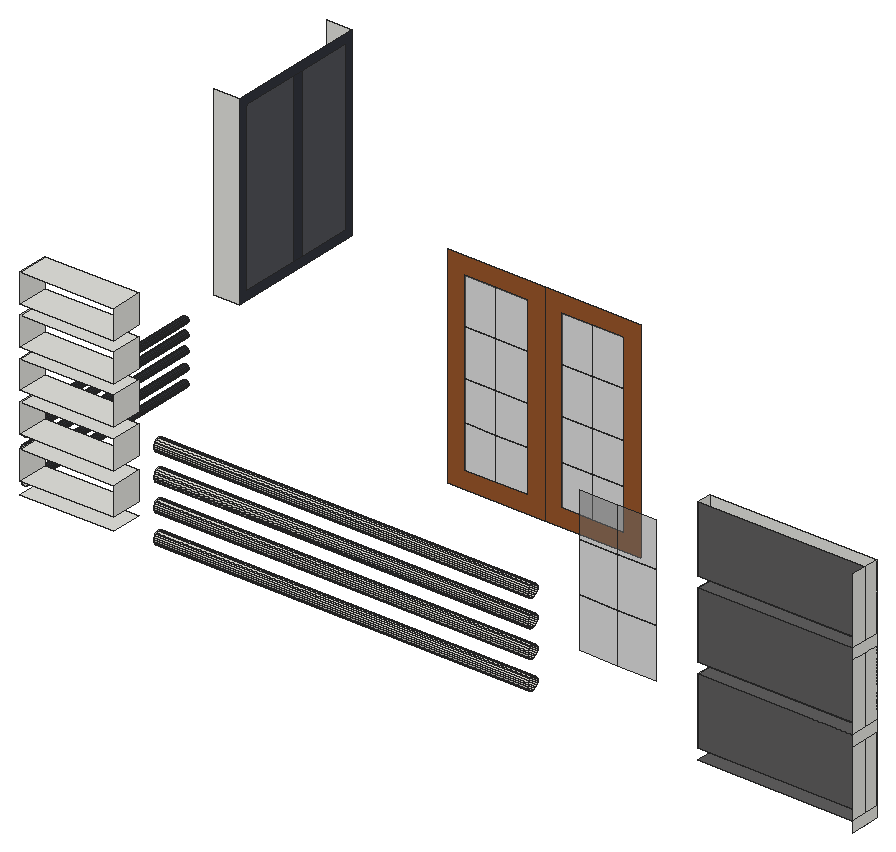
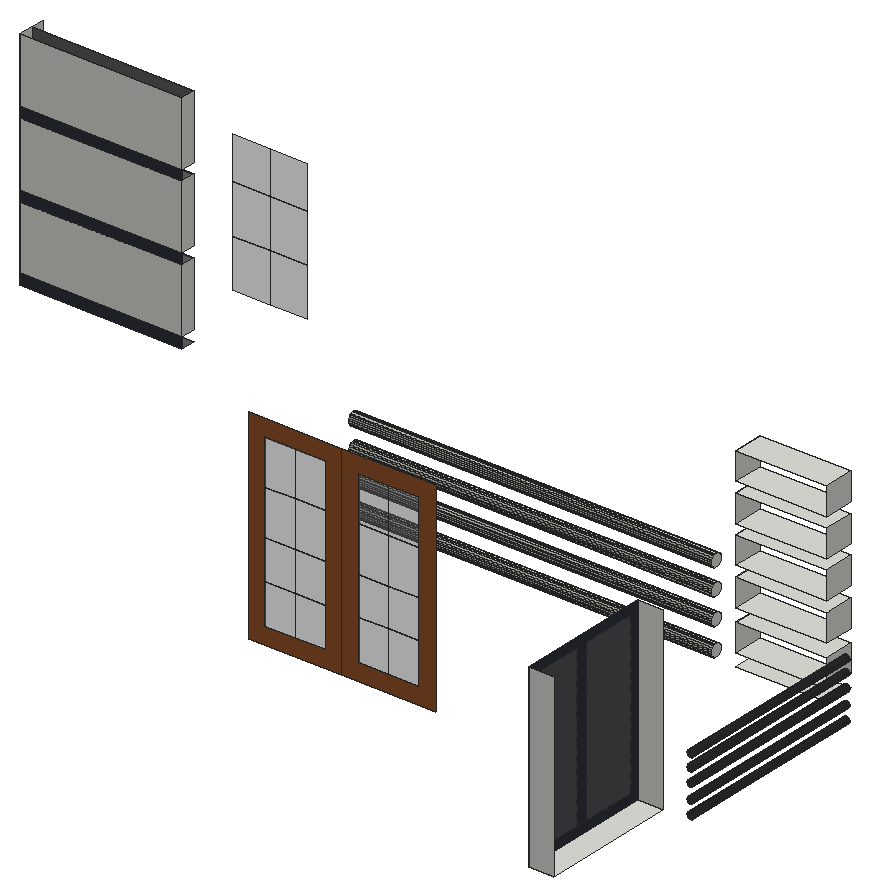
# SketchUp Ruby script. Lengths in inches.
U = 1.inch
M = Sketchup.active_model
def pt(a) = Geom::Point3d.new(a.map { |v| v * U })
def face(e, loops, mat)
  f = e.add_face(loops[0].map { |a| pt(a) })
  loops[1..].each { |l| e.add_face(l.map { |a| pt(a) }).erase! }
  f.material = f.back_material = mat if mat
  f
end
# faces: each face lists its corners as indices into pts; further lists are holes
def faces(e, pts, list, mat = nil) = list.each { |f| face(e, (f[0].is_a?(Array) ? f : [f]).map { |l| l.map { |i| pts[i] } }, mat) }
# xy, xz, yz: faces in a plane at the given z, y or x. An outline is a flat list of corners, or four numbers for a rectangle; further outlines are holes
def ring(l) = l.size == 4 ? [[l[0], l[1]], [l[2], l[1]], [l[2], l[3]], [l[0], l[3]]] : l.each_slice(2).to_a
def flat(e, list, mat, &to3) = list.each { |f| face(e, (f[0].is_a?(Array) ? f : [f]).map { |l| ring(l).map { |u, v| to3.(u, v) } }, mat) }
def xy(e, z, list, mat = nil) = flat(e, list, mat) { |x, y| [x, y, z] }
def xz(e, y, list, mat = nil) = flat(e, list, mat) { |x, z| [x, y, z] }
def yz(e, x, list, mat = nil) = flat(e, list, mat) { |y, z| [x, y, z] }
def lines(e, pts, list) = list.each { |a, b| e.add_line(pt(pts[a]), pt(pts[b])) }
# prism: a flat outline (further loops are holes) pulled along v
def prism(e, loops, v, mat = nil)
  f = face(e, loops, mat); d = Geom::Vector3d.new(v.map { |x| x * U })
  f.pushpull(f.normal.samedirection?(d) ? d.length : -d.length)
end
def box(e, o, s, mat = nil) = prism(e, [[o, [o[0] + s[0], o[1], o[2]], [o[0] + s[0], o[1] + s[1], o[2]], [o[0], o[1] + s[1], o[2]]]], [0, 0, s[2]], mat)
def at(x, y, z, deg = 0) = Geom::Transformation.translation(pt([x, y, z])) * Geom::Transformation.rotation(ORIGIN, Z_AXIS, deg.degrees)
def axes(o, x, y, z) = Geom::Transformation.new([*x, 0, *y, 0, *z, 0, *pt(o).to_a, 1])
def part(name) = M.definitions.add(name)
# library, detail: a bought-in or finely detailed component or shape, given as its bounding box
def library(name, o, s) = part(name).tap { |d| box(d.entities, o, s) }
def detail(e, o, s) = box(e.add_group.entities, o, s)
def put(e, d, t, mat = nil) = e.add_instance(d, t).tap { |i| i.material = mat if mat }
def group(e, t, mat = nil) = e.add_group.tap { |g| g.transformation = t; g.material = mat if mat }.entities
root = M.entities
M.materials.add("[Blinds Roman Hobbled Blue]").color = [81, 82, 87]
M.materials.add("[Formica Laminate Dark]").color = [50, 53, 60]
M.materials.add("[Granite Dark Gray]").color = [96, 95, 95]
M.materials.add("[Terrazzo Tile Light]").color = [219, 217, 210]
M.materials.add("[Translucent Glass Gray]").color = [128, 128, 128]
M.materials["[Translucent Glass Gray]"].alpha = 0.5
M.materials.add("[Wood Cherry Original]").color = [152, 86, 42]
xy(root,221.9,[[23.59,55.96,54.34,66.17]])
xy(root,226.03,[[23.59,55.96,54.34,66.17]])
xy(root,232.83,[[9.125,153.59,17.5,199.9]])
xy(root,235.3125,[[261.16,37.37,315.98,42.24]],"[Granite Dark Gray]")
xy(root,235.4,[[23.59,55.96,54.34,66.17]])
xy(root,238.87,[[261.16,37.37,315.98,42.24]],"[Granite Dark Gray]")
xy(root,239.78,[[23.59,55.96,54.34,66.17]])
xy(root,249.15,[[23.59,55.96,54.34,66.17]])
xy(root,252.65,[[23.59,55.96,54.34,66.17]])
xy(root,260.6875,[[261.16,37.37,315.98,42.24]],"[Granite Dark Gray]")
xy(root,262.03,[[23.59,55.96,54.34,66.17]])
xy(root,264.24,[[261.16,37.37,315.98,42.24]],"[Granite Dark Gray]")
xy(root,265.34,[[23.59,55.96,54.34,66.17]])
xy(root,274.72,[[23.59,55.96,54.34,66.17]])
xy(root,278.15,[[23.59,55.96,54.34,66.17]])
xy(root,286.0625,[[261.16,37.37,315.98,42.24]],"[Granite Dark Gray]")
xy(root,287.53,[[23.59,55.96,54.34,66.17]])
xy(root,289.62,[[261.16,37.37,315.98,42.24]],"[Granite Dark Gray]")
xz(root,36.24,[[223.21,254.56,235.94,271.03],[235.94,254.56,248.67,271.03],[223.21,271.03,235.94,287.51],[235.94,271.03,248.67,287.51],[223.21,287.51,235.94,302.2],
  [235.94,287.51,248.67,302.2]],"[Translucent Glass Gray]")
xz(root,37.37,[[261.16,238.87,315.98,260.6875],[261.16,264.24,315.98,286.0625],[261.16,289.62,315.98,311.4375]],"[Granite Dark Gray]")
xz(root,42.24,[[261.16,238.87,315.98,260.6875],[261.16,264.24,315.98,286.0625],[261.16,289.62,315.98,311.4375]])
xz(root,42.24,[[261.16,235.3125,315.98,238.87],[261.16,260.6875,315.98,264.24],[261.16,286.0625,315.98,289.62]],"[Formica Laminate Dark]")
xz(root,66.17,[[16.85,217.6875,17.15,217.73,17.42,217.84,17.65,218.02,17.83,218.25,17.94,218.52,17.98,218.8125,17.94,219.11,17.83,219.375,17.65,219.61,17.42,219.79,17.15,219.9,16.85,219.9375,16.5625,219.9,16.29,219.79,16.06,219.61,15.88,219.375,15.77,219.11,15.73,218.8125,15.77,218.52,15.88,218.25,16.06,218.02,16.29,217.84,16.5625,217.73],[16.85,222.375,17.15,222.41,17.42,222.53,17.65,222.71,17.83,222.9375,17.94,223.21,17.98,223.5,17.94,223.79,17.83,224.0625,17.65,224.3,17.42,224.48,17.15,224.59,16.85,224.625,16.5625,224.59,16.29,224.48,16.06,224.3,15.88,224.0625,15.77,223.79,15.73,223.5,15.77,223.21,15.88,222.9375,16.06,222.71,16.29,222.53,16.5625,222.41],[16.85,227.5,17.15,227.54,17.42,227.65,17.65,227.83,17.83,228.0625,17.94,228.34,17.98,228.625,17.94,228.92,17.83,229.1875,17.65,229.42,17.42,229.6,17.15,229.71,16.85,229.75,16.5625,229.71,16.29,229.6,16.06,229.42,15.88,229.1875,15.77,228.92,15.73,228.625,15.77,228.34,15.88,228.0625,16.06,227.83,16.29,227.65,16.5625,227.54],[16.85,232.1875,17.15,232.23,17.42,232.34,17.65,232.52,17.83,232.75,17.94,233.02,17.98,233.3125,17.94,233.61,17.83,233.875,17.65,234.11,17.42,234.29,17.15,234.4,16.85,234.4375,16.5625,234.4,16.29,234.29,16.06,234.11,15.88,233.875,15.77,233.61,15.73,233.3125,15.77,233.02,15.88,232.75,16.06,232.52,16.29,232.34,16.5625,232.23],[16.85,236.5,17.15,236.54,17.42,236.65,17.65,236.83,17.83,237.0625,17.94,237.34,17.98,237.625,17.94,237.92,17.83,238.1875,17.65,238.42,17.42,238.6,17.15,238.71,16.85,238.75,16.5625,238.71,16.29,238.6,16.06,238.42,15.88,238.1875,15.77,237.92,15.73,237.625,15.77,237.34,15.88,237.0625,16.06,236.83,16.29,236.65,16.5625,236.54]])
xz(root,132.14,[[108.86,225.54,119.1,239.44],[119.1,225.54,129.35,239.44],[140.51,225.54,150.76,239],[150.76,225.54,161,239],[140.51,239,150.76,252.45],
  [150.76,239,161,252.45],[108.86,239.44,119.1,252.45],[119.1,239.44,129.35,252.45],[108.86,252.45,119.1,267.79],[119.1,252.45,129.35,267.79],
  [140.51,252.45,150.76,267.79],[150.76,252.45,161,267.79],[108.86,267.79,119.1,283.12],[119.1,267.79,129.35,283.12],[140.51,267.79,150.76,283.12],
  [150.76,267.79,161,283.12]],"[Translucent Glass Gray]")
xz(root,132.14,[[[103.27,219.96,134.93,288.7],[108.86,225.54,129.35,283.12]],[[134.93,219.96,166.59,288.7],[140.51,225.54,161,283.12]]],"[Wood Cherry Original]")
xz(root,153.59,[[9.125,232.83,17.5,293.4]])
xz(root,199.9,[[9.125,232.83,17.5,293.4]])
yz(root,17.5,[[156.65,235.9,175.49,290.33],[179.47,235.9,196.84,290.33]],"[Blinds Roman Hobbled Blue]")
yz(root,17.5,[[[153.59,232.83,199.9,293.4],[156.65,235.9,196.84,290.33]],[175.49,235.9,179.47,290.33]],"[Formica Laminate Dark]")
yz(root,23.59,[[55.96,226.03,66.17,235.4],[55.96,239.78,66.17,249.15],[55.96,252.65,66.17,262.03],[55.96,265.34,66.17,274.72],[55.96,278.15,66.17,287.53]])
yz(root,54.34,[[55.96,226.03,66.17,235.4],[55.96,239.78,66.17,249.15],[55.96,252.65,66.17,262.03],[55.96,265.34,66.17,274.72],[55.96,278.15,66.17,287.53]])
yz(root,64.52,[[61.67,219.21,61.14,219.28,60.64,219.48,60.21,219.8125,59.88,220.24,59.68,220.74,59.61,221.27,59.68,221.8,59.88,222.3,60.21,222.73,60.64,223.06,61.14,223.26,61.67,223.33,62.2,223.26,62.7,223.06,63.13,222.73,63.46,222.3,63.66,221.8,63.73,221.27,63.66,220.74,63.46,220.24,63.13,219.8125,62.7,219.48,62.2,219.28],[61.67,228.64,61.14,228.71,60.64,228.92,60.21,229.25,59.88,229.68,59.68,230.17,59.61,230.71,59.68,231.24,59.88,231.74,60.21,232.17,60.64,232.49,61.14,232.7,61.67,232.77,62.2,232.7,62.7,232.49,63.13,232.17,63.46,231.74,63.66,231.24,63.73,230.71,63.66,230.17,63.46,229.68,63.13,229.25,62.7,228.92,62.2,228.71],[61.67,237.71,61.14,237.78,60.64,237.98,60.21,238.3125,59.88,238.74,59.68,239.24,59.61,239.77,59.68,240.3,59.88,240.8,60.21,241.23,60.64,241.56,61.14,241.76,61.67,241.83,62.2,241.76,62.7,241.56,63.13,241.23,63.46,240.8,63.66,240.3,63.73,239.77,63.66,239.24,63.46,238.74,63.13,238.3125,62.7,237.98,62.2,237.78],[61.67,246.58,61.14,246.65,60.64,246.86,60.21,247.1875,59.88,247.61,59.68,248.11,59.61,248.64,59.68,249.18,59.88,249.68,60.21,250.1,60.64,250.43,61.14,250.64,61.67,250.71,62.2,250.64,62.7,250.43,63.13,250.1,63.46,249.68,63.66,249.18,63.73,248.64,63.66,248.11,63.46,247.61,63.13,247.1875,62.7,246.86,62.2,246.65]])
yz(root,261.16,[[37.37,238.87,42.24,260.6875],[37.37,264.24,42.24,286.0625],[37.37,289.62,42.24,311.4375]])
yz(root,315.98,[[32.62,235.3125,42.24,238.87],[32.62,238.87,37.37,260.6875],[37.37,238.87,42.24,260.6875],[32.62,260.6875,42.24,264.24],[32.62,264.24,37.37,286.0625],
  [37.37,264.24,42.24,286.0625],[32.62,286.0625,42.24,289.62],[32.62,289.62,37.37,311.4375],[37.37,289.62,42.24,311.4375]])
p = [[16.5625,66.17,217.73],[16.29,66.17,217.84],[16.29,132.14,217.84],[16.5625,132.14,217.73],[16.85,66.17,217.6875],[16.85,132.14,217.6875],
  [17.15,66.17,217.73],[17.15,132.14,217.73],[17.42,66.17,217.84],[17.42,132.14,217.84],[16.06,66.17,218.02],[16.06,132.14,218.02],
  [17.65,66.17,218.02],[17.65,132.14,218.02],[15.88,66.17,218.25],[15.88,132.14,218.25],[17.83,66.17,218.25],[17.83,132.14,218.25],
  [15.77,66.17,218.52],[15.77,132.14,218.52],[17.94,66.17,218.52],[17.94,132.14,218.52],[15.73,66.17,218.8125],[15.73,132.14,218.8125],
  [17.98,66.17,218.8125],[17.98,132.14,218.8125],[15.77,66.17,219.11],[15.77,132.14,219.11],[17.94,66.17,219.11],[17.94,132.14,219.11],
  [15.88,66.17,219.375],[15.88,132.14,219.375],[17.83,66.17,219.375],[17.83,132.14,219.375],[64.52,61.14,219.28],[64.52,61.67,219.21],
  [187.4,61.67,219.21],[187.4,61.14,219.28],[64.52,62.2,219.28],[187.4,62.2,219.28],[64.52,60.64,219.48],[187.4,60.64,219.48],
  [64.52,62.7,219.48],[187.4,62.7,219.48],[16.06,66.17,219.61],[16.06,132.14,219.61],[17.65,66.17,219.61],[17.65,132.14,219.61],
  [64.52,60.21,219.8125],[187.4,60.21,219.8125],[64.52,63.13,219.8125],[187.4,63.13,219.8125],[16.29,66.17,219.79],[16.29,132.14,219.79],
  [17.42,66.17,219.79],[17.42,132.14,219.79],[64.52,59.88,220.24],[187.4,59.88,220.24],[64.52,63.46,220.24],[187.4,63.46,220.24],
  [16.5625,66.17,219.9],[16.5625,132.14,219.9],[17.15,66.17,219.9],[17.15,132.14,219.9],[16.85,66.17,219.9375],[16.85,132.14,219.9375],
  [64.52,59.68,220.74],[187.4,59.68,220.74],[64.52,63.66,220.74],[187.4,63.66,220.74],[64.52,59.61,221.27],[187.4,59.61,221.27],
  [64.52,63.73,221.27],[187.4,63.73,221.27],[64.52,59.68,221.8],[187.4,59.68,221.8],[64.52,63.66,221.8],[187.4,63.66,221.8],
  [64.52,59.88,222.3],[187.4,59.88,222.3],[64.52,63.46,222.3],[187.4,63.46,222.3],[64.52,60.21,222.73],[187.4,60.21,222.73],
  [64.52,63.13,222.73],[187.4,63.13,222.73],[16.5625,66.17,222.41],[16.29,66.17,222.53],[16.29,132.14,222.53],[16.5625,132.14,222.41],
  [16.85,66.17,222.375],[16.85,132.14,222.375],[17.15,66.17,222.41],[17.15,132.14,222.41],[17.42,66.17,222.53],[17.42,132.14,222.53],
  [16.06,66.17,222.71],[16.06,132.14,222.71],[17.65,66.17,222.71],[17.65,132.14,222.71],[64.52,60.64,223.06],[187.4,60.64,223.06],
  [64.52,62.7,223.06],[187.4,62.7,223.06],[15.88,66.17,222.9375],[15.88,132.14,222.9375],[17.83,66.17,222.9375],[17.83,132.14,222.9375],
  [15.77,66.17,223.21],[15.77,132.14,223.21],[17.94,66.17,223.21],[17.94,132.14,223.21],[64.52,61.14,223.26],[187.4,61.14,223.26],
  [64.52,62.2,223.26],[187.4,62.2,223.26],[15.73,66.17,223.5],[15.73,132.14,223.5],[17.98,66.17,223.5],[17.98,132.14,223.5],
  [64.52,61.67,223.33],[187.4,61.67,223.33],[15.77,66.17,223.79],[15.77,132.14,223.79],[17.94,66.17,223.79],[17.94,132.14,223.79],
  [15.88,66.17,224.0625],[15.88,132.14,224.0625],[17.83,66.17,224.0625],[17.83,132.14,224.0625],[16.06,66.17,224.3],[16.06,132.14,224.3],
  [17.65,66.17,224.3],[17.65,132.14,224.3],[16.29,66.17,224.48],[16.29,132.14,224.48],[17.42,66.17,224.48],[17.42,132.14,224.48],
  [16.5625,66.17,224.59],[16.5625,132.14,224.59],[17.15,66.17,224.59],[17.15,132.14,224.59],[16.85,66.17,224.625],[16.85,132.14,224.625],
  [16.5625,66.17,227.54],[16.29,66.17,227.65],[16.29,132.14,227.65],[16.5625,132.14,227.54],[16.85,66.17,227.5],[16.85,132.14,227.5],
  [17.15,66.17,227.54],[17.15,132.14,227.54],[17.42,66.17,227.65],[17.42,132.14,227.65],[16.06,66.17,227.83],[16.06,132.14,227.83],
  [17.65,66.17,227.83],[17.65,132.14,227.83],[15.88,66.17,228.0625],[15.88,132.14,228.0625],[17.83,66.17,228.0625],[17.83,132.14,228.0625],
  [15.77,66.17,228.34],[15.77,132.14,228.34],[17.94,66.17,228.34],[17.94,132.14,228.34],[15.73,66.17,228.625],[15.73,132.14,228.625],
  [17.98,66.17,228.625],[17.98,132.14,228.625],[64.52,61.14,228.71],[64.52,61.67,228.64],[187.4,61.67,228.64],[187.4,61.14,228.71],
  [64.52,62.2,228.71],[187.4,62.2,228.71],[15.77,66.17,228.92],[15.77,132.14,228.92],[17.94,66.17,228.92],[17.94,132.14,228.92],
  [64.52,60.64,228.92],[187.4,60.64,228.92],[64.52,62.7,228.92],[187.4,62.7,228.92],[64.52,60.21,229.25],[187.4,60.21,229.25],
  [64.52,63.13,229.25],[187.4,63.13,229.25],[15.88,66.17,229.1875],[15.88,132.14,229.1875],[17.83,66.17,229.1875],[17.83,132.14,229.1875],
  [64.52,59.88,229.68],[187.4,59.88,229.68],[64.52,63.46,229.68],[187.4,63.46,229.68],[16.06,66.17,229.42],[16.06,132.14,229.42],
  [17.65,66.17,229.42],[17.65,132.14,229.42],[16.29,66.17,229.6],[16.29,132.14,229.6],[17.42,66.17,229.6],[17.42,132.14,229.6],
  [16.5625,66.17,229.71],[16.5625,132.14,229.71],[17.15,66.17,229.71],[17.15,132.14,229.71],[64.52,59.68,230.17],[187.4,59.68,230.17],
  [64.52,63.66,230.17],[187.4,63.66,230.17],[16.85,66.17,229.75],[16.85,132.14,229.75],[64.52,59.61,230.71],[187.4,59.61,230.71],
  [64.52,63.73,230.71],[187.4,63.73,230.71],[64.52,59.68,231.24],[187.4,59.68,231.24],[64.52,63.66,231.24],[187.4,63.66,231.24],
  [64.52,59.88,231.74],[187.4,59.88,231.74],[64.52,63.46,231.74],[187.4,63.46,231.74],[64.52,60.21,232.17],[187.4,60.21,232.17],
  [64.52,63.13,232.17],[187.4,63.13,232.17],[64.52,60.64,232.49],[187.4,60.64,232.49],[64.52,62.7,232.49],[187.4,62.7,232.49],
  [16.5625,66.17,232.23],[16.29,66.17,232.34],[16.29,132.14,232.34],[16.5625,132.14,232.23],[16.85,66.17,232.1875],[16.85,132.14,232.1875],
  [17.15,66.17,232.23],[17.15,132.14,232.23],[17.42,66.17,232.34],[17.42,132.14,232.34],[16.06,66.17,232.52],[16.06,132.14,232.52],
  [17.65,66.17,232.52],[17.65,132.14,232.52],[64.52,61.14,232.7],[187.4,61.14,232.7],[64.52,62.2,232.7],[187.4,62.2,232.7],
  [15.88,66.17,232.75],[15.88,132.14,232.75],[17.83,66.17,232.75],[17.83,132.14,232.75],[64.52,61.67,232.77],[187.4,61.67,232.77],
  [15.77,66.17,233.02],[15.77,132.14,233.02],[17.94,66.17,233.02],[17.94,132.14,233.02],[15.73,66.17,233.3125],[15.73,132.14,233.3125],
  [17.98,66.17,233.3125],[17.98,132.14,233.3125],[15.77,66.17,233.61],[15.77,132.14,233.61],[17.94,66.17,233.61],[17.94,132.14,233.61],
  [15.88,66.17,233.875],[15.88,132.14,233.875],[17.83,66.17,233.875],[17.83,132.14,233.875],[16.06,66.17,234.11],[16.06,132.14,234.11],
  [17.65,66.17,234.11],[17.65,132.14,234.11],[16.29,66.17,234.29],[16.29,132.14,234.29],[17.42,66.17,234.29],[17.42,132.14,234.29],
  [16.5625,66.17,234.4],[16.5625,132.14,234.4],[17.15,66.17,234.4],[17.15,132.14,234.4],[16.85,66.17,234.4375],[16.85,132.14,234.4375],
  [16.5625,66.17,236.54],[16.29,66.17,236.65],[16.29,132.14,236.65],[16.5625,132.14,236.54],[16.85,66.17,236.5],[16.85,132.14,236.5],
  [17.15,66.17,236.54],[17.15,132.14,236.54],[17.42,66.17,236.65],[17.42,132.14,236.65],[16.06,66.17,236.83],[16.06,132.14,236.83],
  [17.65,66.17,236.83],[17.65,132.14,236.83],[15.88,66.17,237.0625],[15.88,132.14,237.0625],[17.83,66.17,237.0625],[17.83,132.14,237.0625],
  [15.77,66.17,237.34],[15.77,132.14,237.34],[17.94,66.17,237.34],[17.94,132.14,237.34],[15.73,66.17,237.625],[15.73,132.14,237.625],
  [17.98,66.17,237.625],[17.98,132.14,237.625],[15.77,66.17,237.92],[15.77,132.14,237.92],[17.94,66.17,237.92],[17.94,132.14,237.92],
  [64.52,61.14,237.78],[64.52,61.67,237.71],[187.4,61.67,237.71],[187.4,61.14,237.78],[64.52,62.2,237.78],[187.4,62.2,237.78],
  [64.52,60.64,237.98],[187.4,60.64,237.98],[64.52,62.7,237.98],[187.4,62.7,237.98],[15.88,66.17,238.1875],[15.88,132.14,238.1875],
  [17.83,66.17,238.1875],[17.83,132.14,238.1875],[64.52,60.21,238.3125],[187.4,60.21,238.3125],[64.52,63.13,238.3125],[187.4,63.13,238.3125],
  [16.06,66.17,238.42],[16.06,132.14,238.42],[17.65,66.17,238.42],[17.65,132.14,238.42],[64.52,59.88,238.74],[187.4,59.88,238.74],
  [64.52,63.46,238.74],[187.4,63.46,238.74],[16.29,66.17,238.6],[16.29,132.14,238.6],[17.42,66.17,238.6],[17.42,132.14,238.6],
  [16.5625,66.17,238.71],[16.5625,132.14,238.71],[17.15,66.17,238.71],[17.15,132.14,238.71],[64.52,59.68,239.24],[187.4,59.68,239.24],
  [64.52,63.66,239.24],[187.4,63.66,239.24],[16.85,66.17,238.75],[16.85,132.14,238.75],[64.52,59.61,239.77],[187.4,59.61,239.77],
  [64.52,63.73,239.77],[187.4,63.73,239.77],[64.52,59.68,240.3],[187.4,59.68,240.3],[64.52,63.66,240.3],[187.4,63.66,240.3],
  [64.52,59.88,240.8],[187.4,59.88,240.8],[64.52,63.46,240.8],[187.4,63.46,240.8],[64.52,60.21,241.23],[187.4,60.21,241.23],
  [64.52,63.13,241.23],[187.4,63.13,241.23],[64.52,60.64,241.56],[187.4,60.64,241.56],[64.52,62.7,241.56],[187.4,62.7,241.56],
  [64.52,61.14,241.76],[187.4,61.14,241.76],[64.52,62.2,241.76],[187.4,62.2,241.76],[64.52,61.67,241.83],[187.4,61.67,241.83],
  [64.52,61.14,246.65],[64.52,61.67,246.58],[187.4,61.67,246.58],[187.4,61.14,246.65],[64.52,62.2,246.65],[187.4,62.2,246.65],
  [64.52,60.64,246.86],[187.4,60.64,246.86],[64.52,62.7,246.86],[187.4,62.7,246.86],[64.52,60.21,247.1875],[187.4,60.21,247.1875],
  [64.52,63.13,247.1875],[187.4,63.13,247.1875],[64.52,59.88,247.61],[187.4,59.88,247.61],[64.52,63.46,247.61],[187.4,63.46,247.61],
  [64.52,59.68,248.11],[187.4,59.68,248.11],[64.52,63.66,248.11],[187.4,63.66,248.11],[64.52,59.61,248.64],[187.4,59.61,248.64],
  [64.52,63.73,248.64],[187.4,63.73,248.64],[64.52,59.68,249.18],[187.4,59.68,249.18],[64.52,63.66,249.18],[187.4,63.66,249.18],
  [64.52,59.88,249.68],[187.4,59.88,249.68],[64.52,63.46,249.68],[187.4,63.46,249.68],[64.52,60.21,250.1],[187.4,60.21,250.1],
  [64.52,63.13,250.1],[187.4,63.13,250.1],[64.52,60.64,250.43],[187.4,60.64,250.43],[64.52,62.7,250.43],[187.4,62.7,250.43],
  [64.52,61.14,250.64],[187.4,61.14,250.64],[64.52,62.2,250.64],[187.4,62.2,250.64],[64.52,61.67,250.71],[187.4,61.67,250.71]]
faces(root,p,[[0,1,2,3],[4,0,3,5],[6,4,5,7],[8,6,7,9],[1,10,11,2],[12,8,9,13],[10,14,15,11],[16,12,13,17],
  [14,18,19,15],[20,16,17,21],[18,22,23,19],[24,20,21,25],[22,26,27,23],[28,24,25,29],[26,30,31,27],[32,28,29,33],
  [30,44,45,31],[46,32,33,47],[44,52,53,45],[54,46,47,55],[52,60,61,53],[62,54,55,63],[60,64,65,61],[64,62,63,65],
  [86,87,88,89],[90,86,89,91],[92,90,91,93],[94,92,93,95],[87,96,97,88],[98,94,95,99],[96,104,105,97],[106,98,99,107],
  [104,108,109,105],[110,106,107,111],[108,116,117,109],[118,110,111,119],[116,122,123,117],[124,118,119,125],[122,126,127,123],[128,124,125,129],
  [126,130,131,127],[132,128,129,133],[130,134,135,131],[136,132,133,137],[134,138,139,135],[140,136,137,141],[138,142,143,139],[142,140,141,143],
  [144,145,146,147],[148,144,147,149],[150,148,149,151],[152,150,151,153],[145,154,155,146],[156,152,153,157],[154,158,159,155],[160,156,157,161],
  [158,162,163,159],[164,160,161,165],[162,166,167,163],[168,164,165,169],[166,176,177,167],[178,168,169,179],[176,188,189,177],[190,178,179,191],
  [188,196,197,189],[198,190,191,199],[196,200,201,197],[202,198,199,203],[200,204,205,201],[206,202,203,207],[204,212,213,205],[212,206,207,213],
  [234,235,236,237],[238,234,237,239],[240,238,239,241],[242,240,241,243],[235,244,245,236],[246,242,243,247],[244,252,253,245],[254,246,247,255],
  [252,258,259,253],[260,254,255,261],[258,262,263,259],[264,260,261,265],[262,266,267,263],[268,264,265,269],[266,270,271,267],[272,268,269,273],
  [270,274,275,271],[276,272,273,277],[274,278,279,275],[280,276,277,281],[278,282,283,279],[284,280,281,285],[282,286,287,283],[286,284,285,287],
  [288,289,290,291],[292,288,291,293],[294,292,293,295],[296,294,295,297],[289,298,299,290],[300,296,297,301],[298,302,303,299],[304,300,301,305],
  [302,306,307,303],[308,304,305,309],[306,310,311,307],[312,308,309,313],[310,314,315,311],[316,312,313,317],[314,328,329,315],[330,316,317,331],
  [328,336,337,329],[338,330,331,339],[336,344,345,337],[346,338,339,347],[344,348,349,345],[350,346,347,351],[348,356,357,349],[356,350,351,357]],"[Formica Laminate Dark]")
faces(root,p,[[34,35,36,37],[35,38,39,36],[40,34,37,41],[38,42,43,39],[48,40,41,49],[42,50,51,43],[56,48,49,57],[50,58,59,51],
  [66,56,57,67],[58,68,69,59],[70,66,67,71],[68,72,73,69],[74,70,71,75],[72,76,77,73],[78,74,75,79],[76,80,81,77],
  [82,78,79,83],[80,84,85,81],[100,82,83,101],[84,102,103,85],[112,100,101,113],[102,114,115,103],[120,112,113,121],[114,120,121,115],
  [170,171,172,173],[171,174,175,172],[180,170,173,181],[174,182,183,175],[184,180,181,185],[182,186,187,183],[192,184,185,193],[186,194,195,187],
  [208,192,193,209],[194,210,211,195],[214,208,209,215],[210,216,217,211],[218,214,215,219],[216,220,221,217],[222,218,219,223],[220,224,225,221],
  [226,222,223,227],[224,228,229,225],[230,226,227,231],[228,232,233,229],[248,230,231,249],[232,250,251,233],[256,248,249,257],[250,256,257,251],
  [318,319,320,321],[319,322,323,320],[324,318,321,325],[322,326,327,323],[332,324,325,333],[326,334,335,327],[340,332,333,341],[334,342,343,335],
  [352,340,341,353],[342,354,355,343],[358,352,353,359],[354,360,361,355],[362,358,359,363],[360,364,365,361],[366,362,363,367],[364,368,369,365],
  [370,366,367,371],[368,372,373,369],[374,370,371,375],[372,376,377,373],[378,374,375,379],[376,380,381,377],[382,378,379,383],[380,382,383,381],
  [384,385,386,387],[385,388,389,386],[390,384,387,391],[388,392,393,389],[394,390,391,395],[392,396,397,393],[398,394,395,399],[396,400,401,397],
  [402,398,399,403],[400,404,405,401],[406,402,403,407],[404,408,409,405],[410,406,407,411],[408,412,413,409],[414,410,411,415],[412,416,417,413],
  [418,414,415,419],[416,420,421,417],[422,418,419,423],[420,424,425,421],[426,422,423,427],[424,428,429,425],[430,426,427,431],[428,430,431,429]],"[Terrazzo Tile Light]")
